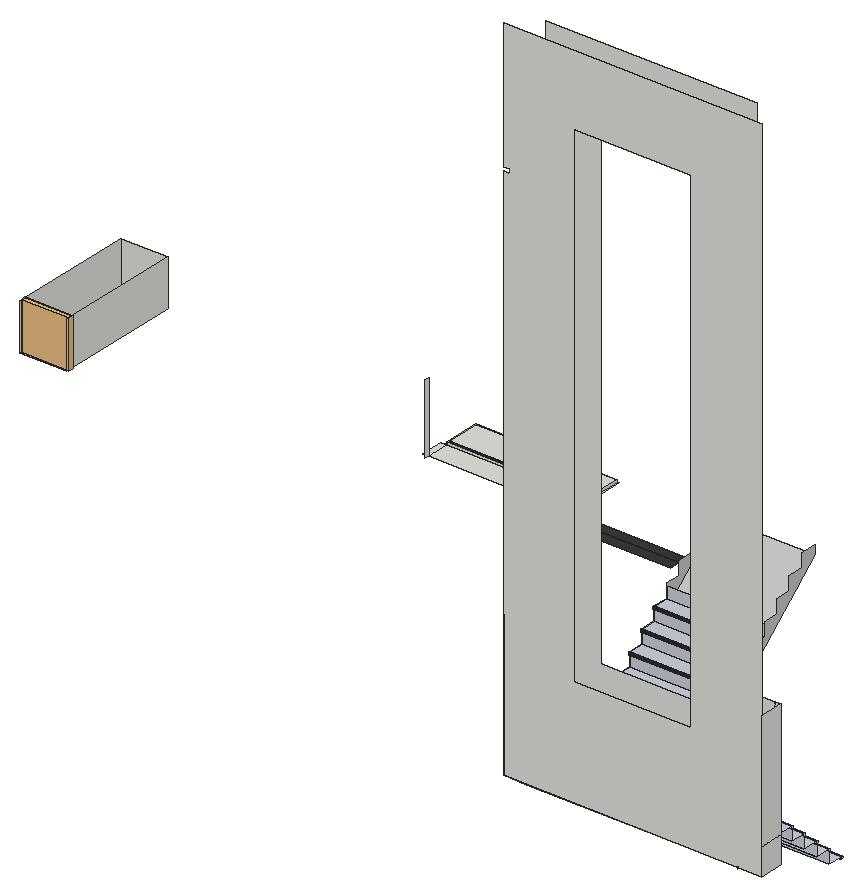
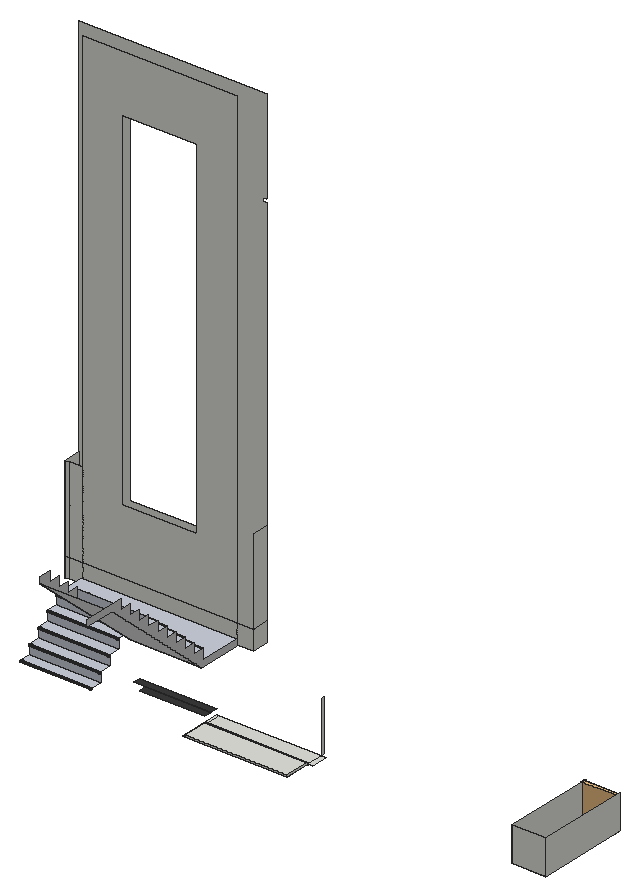
# SketchUp Ruby script. Lengths in inches.
U = 1.inch
M = Sketchup.active_model
def pt(a) = Geom::Point3d.new(a.map { |v| v * U })
def face(e, loops, mat)
  f = e.add_face(loops[0].map { |a| pt(a) })
  loops[1..].each { |l| e.add_face(l.map { |a| pt(a) }).erase! }
  f.material = f.back_material = mat if mat
  f
end
# faces: each face lists its corners as indices into pts; further lists are holes
def faces(e, pts, list, mat = nil) = list.each { |f| face(e, (f[0].is_a?(Array) ? f : [f]).map { |l| l.map { |i| pts[i] } }, mat) }
# xy, xz, yz: faces in a plane at the given z, y or x. An outline is a flat list of corners, or four numbers for a rectangle; further outlines are holes
def ring(l) = l.size == 4 ? [[l[0], l[1]], [l[2], l[1]], [l[2], l[3]], [l[0], l[3]]] : l.each_slice(2).to_a
def flat(e, list, mat, &to3) = list.each { |f| face(e, (f[0].is_a?(Array) ? f : [f]).map { |l| ring(l).map { |u, v| to3.(u, v) } }, mat) }
def xy(e, z, list, mat = nil) = flat(e, list, mat) { |x, y| [x, y, z] }
def xz(e, y, list, mat = nil) = flat(e, list, mat) { |x, z| [x, y, z] }
def yz(e, x, list, mat = nil) = flat(e, list, mat) { |y, z| [x, y, z] }
def lines(e, pts, list) = list.each { |a, b| e.add_line(pt(pts[a]), pt(pts[b])) }
# prism: a flat outline (further loops are holes) pulled along v
def prism(e, loops, v, mat = nil)
  f = face(e, loops, mat); d = Geom::Vector3d.new(v.map { |x| x * U })
  f.pushpull(f.normal.samedirection?(d) ? d.length : -d.length)
end
def box(e, o, s, mat = nil) = prism(e, [[o, [o[0] + s[0], o[1], o[2]], [o[0] + s[0], o[1] + s[1], o[2]], [o[0], o[1] + s[1], o[2]]]], [0, 0, s[2]], mat)
def at(x, y, z, deg = 0) = Geom::Transformation.translation(pt([x, y, z])) * Geom::Transformation.rotation(ORIGIN, Z_AXIS, deg.degrees)
def axes(o, x, y, z) = Geom::Transformation.new([*x, 0, *y, 0, *z, 0, *pt(o).to_a, 1])
def part(name) = M.definitions.add(name)
# library, detail: a bought-in or finely detailed component or shape, given as its bounding box
def library(name, o, s) = part(name).tap { |d| box(d.entities, o, s) }
def detail(e, o, s) = box(e.add_group.entities, o, s)
def put(e, d, t, mat = nil) = e.add_instance(d, t).tap { |i| i.material = mat if mat }
def group(e, t, mat = nil) = e.add_group.tap { |g| g.transformation = t; g.material = mat if mat }.entities
root = M.entities
M.materials.add("[Color M07]").color = [58, 58, 58]
M.materials.add("[Marble Carrara Floor Tile]").color = [204, 208, 219]
M.materials.add("[Polished Concrete New]").color = [200, 200, 203]
c1 = library("Group\#44",[0,0,0],[24.41,3.15,28.35])
xy(root,45.24,[[417.96,89.93,468,90.26]],"[Marble Carrara Floor Tile]")
xy(root,46.4,[[417.96,82.01,468,89.93],[417.96,89.93,468,90.26]],"[Marble Carrara Floor Tile]")
xy(root,52.21,[[417.96,82.01,468,82.34]],"[Marble Carrara Floor Tile]")
xy(root,53.375,[[417.96,74.09,468,82.01],[417.96,82.01,468,82.34]],"[Marble Carrara Floor Tile]")
xy(root,59.18,[[417.96,74.09,468,74.42]],"[Marble Carrara Floor Tile]")
xy(root,60.34,[[417.96,66.17,468,74.09],[417.96,74.09,468,74.42]],"[Marble Carrara Floor Tile]")
xy(root,66.15,[[417.96,66.17,468,66.5]],"[Marble Carrara Floor Tile]")
xy(root,67.32,[[417.96,58.25,468,66.17],[417.96,66.17,468,66.5]],"[Marble Carrara Floor Tile]")
xy(root,69.71,[[359.58,34.49,359.58,66.78,409.62,66.78,409.62,58.25,417.96,58.25,417.96,49.71,468,49.71,468,34.49]],"[Polished Concrete New]")
xy(root,70.4375,[[348,24,360,36],[360,24,468,36],[468,24,477.125,36],[477.125,24,480,36]])
xy(root,73.125,[[417.96,58.25,468,58.58]],"[Marble Carrara Floor Tile]")
xy(root,74.29,[[359.58,34.49,468,34.49,468,58.25,409.62,58.25,409.62,66.17,359.58,66.17],[417.96,58.25,468,58.58]],"[Marble Carrara Floor Tile]")
xy(root,80.1,[[359.58,65.84,409.62,66.17]],"[Marble Carrara Floor Tile]")
xy(root,81.26,[[359.58,65.84,409.62,66.17],[359.58,66.17,409.62,74.09]],"[Marble Carrara Floor Tile]")
xy(root,87.07,[[359.58,73.76,409.62,74.09]],"[Marble Carrara Floor Tile]")
xy(root,88.23,[[359.58,73.76,409.62,74.09],[359.58,74.09,409.62,82.01]],"[Marble Carrara Floor Tile]")
xy(root,94.04,[[359.58,81.68,409.62,82.01]],"[Marble Carrara Floor Tile]")
xy(root,95.2,[[359.58,81.68,409.62,82.01],[359.58,82.01,409.62,89.93]],"[Marble Carrara Floor Tile]")
xy(root,101.01,[[359.58,89.6,409.62,89.93]],"[Marble Carrara Floor Tile]")
xy(root,102.17,[[359.58,89.6,409.62,89.93],[359.58,89.93,409.62,97.85]],"[Marble Carrara Floor Tile]")
xy(root,104,[[286,151,332,156]],"[Color M07]")
xy(root,107.98,[[359.58,97.52,409.62,97.85]],"[Marble Carrara Floor Tile]")
xy(root,108,[[24,120,48,184.5625],[200.9375,156,204,168],[204,156,276,168],[276,156,277.375,168],[203.375,168,204,169.0625],
  [204,168,276,169.0625],[276,168,276.25,169.0625],[203.8125,169.0625,204,186.3125],[204,169.0625,276,186.3125],[276,169.0625,277.1875,186.3125]])
xy(root,108,[[282,151,336,156]],"[Color M07]")
xy(root,109.125,[[204,168,276,169.0625]])
xy(root,109.14,[[359.58,97.52,409.62,97.85],[359.58,97.85,409.62,105.77]],"[Marble Carrara Floor Tile]")
xy(root,109.375,[[204,169.0625,276,186.3125]])
xy(root,114.95,[[359.58,105.4375,409.62,105.77]],"[Marble Carrara Floor Tile]")
xy(root,116.11,[[359.58,105.4375,409.62,105.77],[359.58,105.77,409.62,113.6875]],"[Marble Carrara Floor Tile]")
xz(root,24,[[[348,70.4375,480,70.4375,480,415.2,348,415.2,348,349.2,351,349.2,351,347.2,348,347.2],[384,126,444,379.2]]])
xz(root,34.49,[[359.58,69.71,468,74.29]],"[Polished Concrete New]")
xz(root,36,[[348,70.4375,360,84],[360,70.4375,468,84],[468,70.4375,477.125,84],[477.125,70.4375,480,84],[[360,84,468,415.2],[388,130,440,375.2]],
  [468,84,477.125,144],[477.125,84,480,144]])
xz(root,58.25,[[417.96,67.32,468,73.125],[417.96,73.125,468,74.29]],"[Marble Carrara Floor Tile]")
xz(root,58.25,[[409.62,69.71,417.96,74.29]],"[Polished Concrete New]")
xz(root,66.17,[[417.96,60.34,468,66.15],[417.96,66.15,468,67.32],[359.58,74.29,409.62,80.1],[359.58,80.1,409.62,81.26]],"[Marble Carrara Floor Tile]")
xz(root,74.09,[[417.96,53.375,468,59.18],[417.96,59.18,468,60.34],[359.58,81.26,409.62,87.07],[359.58,87.07,409.62,88.23]],"[Marble Carrara Floor Tile]")
xz(root,82.01,[[417.96,46.4,468,52.21],[417.96,52.21,468,53.375],[359.58,88.23,409.62,94.04],[359.58,94.04,409.62,95.2]],"[Marble Carrara Floor Tile]")
xz(root,89.93,[[417.96,45.24,468,46.4],[359.58,95.2,409.62,101.01],[359.58,101.01,409.62,102.17]],"[Marble Carrara Floor Tile]")
xz(root,97.85,[[359.58,102.17,409.62,107.98],[359.58,107.98,409.62,109.14]],"[Marble Carrara Floor Tile]")
xz(root,105.77,[[359.58,109.14,409.62,114.95],[359.58,114.95,409.62,116.11]],"[Marble Carrara Floor Tile]")
xz(root,113.6875,[[359.58,116.11,409.62,121.92]],"[Marble Carrara Floor Tile]")
xz(root,168,[[204,108,276,109.125]])
xz(root,169.0625,[[204,108,276,109.125],[204,109.125,276,109.375]])
xz(root,184.5625,[[24,108,48,132]])
xz(root,186.3125,[[204,108,276,109.375]])
yz(root,24,[[120,108,184.5625,132]])
yz(root,48,[[120,108,184.5625,132]])
yz(root,204,[[153.875,108,156,144],[168,108,169.0625,109.125],[169.0625,108,186.3125,109.375]])
yz(root,276,[[168,108,169.0625,109.125],[169.0625,108,186.3125,109.375]])
yz(root,348,[[24,70.4375,36,84],[24,84,36,144]])
yz(root,359.58,[[65.84,80.1,65.75,80.12,65.67,80.17,65.6,80.27,65.55,80.39,65.52,80.53,65.51,80.68,65.52,80.83,65.55,80.97,65.6,81.09,65.67,81.18,65.75,81.24,65.84,81.26,66.17,81.26,66.17,80.1],[73.76,87.07,73.67,87.09,73.59,87.15,73.52,87.24,73.47,87.36,73.4375,87.5,73.43,87.65,73.4375,87.8,73.47,87.9375,73.52,88.06,73.59,88.15,73.67,88.21,73.76,88.23,74.09,88.23,74.09,87.07],[81.68,94.04,81.59,94.06,81.51,94.12,81.44,94.21,81.39,94.33,81.36,94.47,81.35,94.62,81.36,94.77,81.39,94.91,81.44,95.03,81.51,95.125,81.59,95.18,81.68,95.2,82.01,95.2,82.01,94.04],[89.6,101.01,89.51,101.03,89.43,101.09,89.36,101.18,89.31,101.3,89.28,101.44,89.27,101.59,89.28,101.74,89.31,101.88,89.36,102,89.43,102.09,89.51,102.15,89.6,102.17,89.93,102.17,89.93,101.01],[97.52,107.98,97.43,108,97.35,108.06,97.28,108.15,97.23,108.27,97.2,108.41,97.1875,108.5625,97.2,108.71,97.23,108.85,97.28,108.97,97.35,109.07,97.43,109.125,97.52,109.14,97.85,109.14,97.85,107.98],
  [105.4375,114.95,105.35,114.97,105.27,115.03,105.2,115.125,105.15,115.24,105.12,115.38,105.11,115.53,105.12,115.68,105.15,115.82,105.2,115.94,105.27,116.04,105.35,116.1,105.4375,116.11,105.77,116.11,105.77,114.95]],"[Marble Carrara Floor Tile]")
yz(root,359.58,[[34.49,69.71,34.49,74.29,66.17,74.29,66.17,81.26,74.09,81.26,74.09,88.23,82.01,88.23,82.01,95.2,89.93,95.2,89.93,102.17,97.85,102.17,97.85,109.14,105.77,109.14,105.77,116.11,113.6875,116.11,113.6875,123.09,121.61,123.09,121.61,130.06,129.53,130.06,129.53,137.03,137.45,137.03,137.45,144,168,144,168,139.43,145.98,139.43,66.78,69.71]],"[Polished Concrete New]")
yz(root,409.62,[[65.84,80.1,66.17,80.1,66.17,81.26,65.84,81.26,65.75,81.24,65.67,81.18,65.6,81.09,65.55,80.97,65.52,80.83,65.51,80.68,65.52,80.53,65.55,80.39,65.6,80.27,65.67,80.17,65.75,80.12],[73.76,87.07,74.09,87.07,74.09,88.23,73.76,88.23,73.67,88.21,73.59,88.15,73.52,88.06,73.47,87.9375,73.4375,87.8,73.43,87.65,73.4375,87.5,73.47,87.36,73.52,87.24,73.59,87.15,73.67,87.09],[81.68,94.04,82.01,94.04,82.01,95.2,81.68,95.2,81.59,95.18,81.51,95.125,81.44,95.03,81.39,94.91,81.36,94.77,81.35,94.62,81.36,94.47,81.39,94.33,81.44,94.21,81.51,94.12,81.59,94.06],[89.6,101.01,89.93,101.01,89.93,102.17,89.6,102.17,89.51,102.15,89.43,102.09,89.36,102,89.31,101.88,89.28,101.74,89.27,101.59,89.28,101.44,89.31,101.3,89.36,101.18,89.43,101.09,89.51,101.03],[97.52,107.98,97.85,107.98,97.85,109.14,97.52,109.14,97.43,109.125,97.35,109.07,97.28,108.97,97.23,108.85,97.2,108.71,97.1875,108.5625,97.2,108.41,97.23,108.27,97.28,108.15,97.35,108.06,97.43,108],
  [105.4375,114.95,105.77,114.95,105.77,116.11,105.4375,116.11,105.35,116.1,105.27,116.04,105.2,115.94,105.15,115.82,105.12,115.68,105.11,115.53,105.12,115.38,105.15,115.24,105.2,115.125,105.27,115.03,105.35,114.97]],"[Marble Carrara Floor Tile]")
yz(root,409.62,[[58.25,69.71,66.78,69.71,145.98,139.43,145.98,144,137.45,144,137.45,137.03,129.53,137.03,129.53,130.06,121.61,130.06,121.61,123.09,113.6875,123.09,113.6875,116.11,105.77,116.11,105.77,109.14,97.85,109.14,97.85,102.17,89.93,102.17,89.93,95.2,82.01,95.2,82.01,88.23,74.09,88.23,74.09,81.26,66.17,81.26,66.17,74.29,58.25,74.29]],"[Polished Concrete New]")
yz(root,417.96,[[89.93,45.24,89.93,46.4,90.26,46.4,90.34,46.38,90.42,46.32,90.49,46.23,90.54,46.11,90.57,45.97,90.59,45.82,90.57,45.67,90.54,45.53,90.49,45.41,90.42,45.32,90.34,45.26,90.26,45.24],[82.01,52.21,82.01,53.375,82.34,53.375,82.42,53.35,82.5,53.3,82.57,53.2,82.62,53.08,82.65,52.94,82.67,52.79,82.65,52.64,82.62,52.5,82.57,52.38,82.5,52.29,82.42,52.23,82.34,52.21],[74.09,59.18,74.09,60.34,74.42,60.34,74.5,60.32,74.58,60.27,74.65,60.17,74.7,60.05,74.73,59.91,74.75,59.76,74.73,59.61,74.7,59.47,74.65,59.35,74.58,59.26,74.5,59.2,74.42,59.18],[66.17,66.15,66.17,67.32,66.5,67.32,66.58,67.3,66.66,67.24,66.73,67.15,66.78,67.03,66.8125,66.89,66.83,66.73,66.8125,66.58,66.78,66.44,66.73,66.32,66.66,66.23,66.58,66.17,66.5,66.15],[58.25,73.125,58.25,74.29,58.58,74.29,58.66,74.27,58.74,74.21,58.81,74.12,58.86,74,58.89,73.86,58.91,73.71,58.89,73.56,58.86,73.42,58.81,73.3,58.74,73.2,58.66,73.15,58.58,73.125]],"[Marble Carrara Floor Tile]")
yz(root,468,[[24,69.71,34.49,70.4375],[34.49,70.4375,36,74.29]])
yz(root,468,[[89.93,45.24,89.93,46.4,90.26,46.4,90.34,46.38,90.42,46.32,90.49,46.23,90.54,46.11,90.57,45.97,90.59,45.82,90.57,45.67,90.54,45.53,90.49,45.41,90.42,45.32,90.34,45.26,90.26,45.24],[82.01,52.21,82.01,53.375,82.34,53.375,82.42,53.35,82.5,53.3,82.57,53.2,82.62,53.08,82.65,52.94,82.67,52.79,82.65,52.64,82.62,52.5,82.57,52.38,82.5,52.29,82.42,52.23,82.34,52.21],[74.09,59.18,74.09,60.34,74.42,60.34,74.5,60.32,74.58,60.27,74.65,60.17,74.7,60.05,74.73,59.91,74.75,59.76,74.73,59.61,74.7,59.47,74.65,59.35,74.58,59.26,74.5,59.2,74.42,59.18],[66.17,66.15,66.17,67.32,66.5,67.32,66.58,67.3,66.66,67.24,66.73,67.15,66.78,67.03,66.8125,66.89,66.83,66.73,66.8125,66.58,66.78,66.44,66.73,66.32,66.66,66.23,66.58,66.17,66.5,66.15],[58.25,73.125,58.25,74.29,58.58,74.29,58.66,74.27,58.74,74.21,58.81,74.12,58.86,74,58.89,73.86,58.91,73.71,58.89,73.56,58.86,73.42,58.81,73.3,58.74,73.2,58.66,73.15,58.58,73.125]],"[Marble Carrara Floor Tile]")
yz(root,480,[[24,70.4375,36,84],[24,84,36,144]])
p = [[468,90.34,45.26],[468,90.26,45.24],[417.96,90.26,45.24],[417.96,90.34,45.26],[468,90.42,45.32],[417.96,90.42,45.32],
  [468,90.49,45.41],[417.96,90.49,45.41],[468,90.54,45.53],[417.96,90.54,45.53],[468,90.57,45.67],[417.96,90.57,45.67],
  [468,90.59,45.82],[417.96,90.59,45.82],[468,90.57,45.97],[417.96,90.57,45.97],[468,90.54,46.11],[417.96,90.54,46.11],
  [468,90.49,46.23],[417.96,90.49,46.23],[468,90.42,46.32],[417.96,90.42,46.32],[468,90.34,46.38],[417.96,90.34,46.38],
  [468,90.26,46.4],[417.96,90.26,46.4],[468,82.42,52.23],[468,82.34,52.21],[417.96,82.34,52.21],[417.96,82.42,52.23],
  [468,82.5,52.29],[417.96,82.5,52.29],[468,82.57,52.38],[417.96,82.57,52.38],[468,82.62,52.5],[417.96,82.62,52.5],
  [468,82.65,52.64],[417.96,82.65,52.64],[468,82.67,52.79],[417.96,82.67,52.79],[468,82.65,52.94],[417.96,82.65,52.94],
  [468,82.62,53.08],[417.96,82.62,53.08],[468,82.57,53.2],[417.96,82.57,53.2],[468,82.5,53.3],[417.96,82.5,53.3],
  [468,82.42,53.35],[417.96,82.42,53.35],[468,82.34,53.375],[417.96,82.34,53.375],[468,74.5,59.2],[468,74.42,59.18],
  [417.96,74.42,59.18],[417.96,74.5,59.2],[468,74.58,59.26],[417.96,74.58,59.26],[468,74.65,59.35],[417.96,74.65,59.35],
  [468,74.7,59.47],[417.96,74.7,59.47],[468,74.73,59.61],[417.96,74.73,59.61],[468,74.75,59.76],[417.96,74.75,59.76],
  [468,74.73,59.91],[417.96,74.73,59.91],[468,74.7,60.05],[417.96,74.7,60.05],[468,74.65,60.17],[417.96,74.65,60.17],
  [468,74.58,60.27],[417.96,74.58,60.27],[468,74.42,60.34],[468,74.5,60.32],[417.96,74.5,60.32],[417.96,74.42,60.34],
  [468,66.58,66.17],[468,66.5,66.15],[417.96,66.5,66.15],[417.96,66.58,66.17],[468,66.66,66.23],[417.96,66.66,66.23],
  [468,66.73,66.32],[417.96,66.73,66.32],[468,66.78,66.44],[417.96,66.78,66.44],[468,66.8125,66.58],[417.96,66.8125,66.58],
  [468,66.83,66.73],[417.96,66.83,66.73],[468,66.8125,66.89],[417.96,66.8125,66.89],[468,66.78,67.03],[417.96,66.78,67.03],
  [468,66.73,67.15],[417.96,66.73,67.15],[468,66.66,67.24],[417.96,66.66,67.24],[468,66.58,67.3],[417.96,66.58,67.3],
  [468,66.5,67.32],[417.96,66.5,67.32],[359.58,66.78,69.71],[359.58,145.98,139.43],[409.62,145.98,139.43],[409.62,66.78,69.71],
  [468,58.66,73.15],[468,58.58,73.125],[417.96,58.58,73.125],[417.96,58.66,73.15],[468,58.74,73.2],[417.96,58.74,73.2],
  [468,58.81,73.3],[417.96,58.81,73.3],[468,58.86,73.42],[417.96,58.86,73.42],[468,58.89,73.56],[417.96,58.89,73.56],
  [468,58.91,73.71],[417.96,58.91,73.71],[468,58.89,73.86],[417.96,58.89,73.86],[468,58.86,74],[417.96,58.86,74],
  [468,58.81,74.12],[417.96,58.81,74.12],[468,58.74,74.21],[417.96,58.74,74.21],[468,58.66,74.27],[417.96,58.66,74.27],
  [468,58.58,74.29],[417.96,58.58,74.29],[359.58,65.67,80.17],[359.58,65.75,80.12],[409.62,65.75,80.12],[409.62,65.67,80.17],
  [359.58,65.84,80.1],[409.62,65.84,80.1],[359.58,65.6,80.27],[409.62,65.6,80.27],[359.58,65.55,80.39],[409.62,65.55,80.39],
  [359.58,65.52,80.53],[409.62,65.52,80.53],[359.58,65.51,80.68],[409.62,65.51,80.68],[359.58,65.52,80.83],[409.62,65.52,80.83],
  [359.58,65.55,80.97],[409.62,65.55,80.97],[359.58,65.6,81.09],[409.62,65.6,81.09],[359.58,65.67,81.18],[409.62,65.67,81.18],
  [359.58,65.75,81.24],[409.62,65.75,81.24],[359.58,65.84,81.26],[409.62,65.84,81.26],[359.58,73.52,87.24],[359.58,73.59,87.15],
  [409.62,73.59,87.15],[409.62,73.52,87.24],[359.58,73.67,87.09],[409.62,73.67,87.09],[359.58,73.76,87.07],[409.62,73.76,87.07],
  [359.58,73.47,87.36],[409.62,73.47,87.36],[359.58,73.4375,87.5],[409.62,73.4375,87.5],[359.58,73.43,87.65],[409.62,73.43,87.65],
  [359.58,73.4375,87.8],[409.62,73.4375,87.8],[359.58,73.47,87.9375],[409.62,73.47,87.9375],[359.58,73.52,88.06],[409.62,73.52,88.06],
  [359.58,73.59,88.15],[409.62,73.59,88.15],[359.58,73.67,88.21],[409.62,73.67,88.21],[359.58,73.76,88.23],[409.62,73.76,88.23],
  [359.58,81.59,94.06],[359.58,81.68,94.04],[409.62,81.68,94.04],[409.62,81.59,94.06],[359.58,81.44,94.21],[359.58,81.51,94.12],
  [409.62,81.51,94.12],[409.62,81.44,94.21],[359.58,81.39,94.33],[409.62,81.39,94.33],[359.58,81.36,94.47],[409.62,81.36,94.47],
  [359.58,81.35,94.62],[409.62,81.35,94.62],[359.58,81.36,94.77],[409.62,81.36,94.77],[359.58,81.39,94.91],[409.62,81.39,94.91],
  [359.58,81.44,95.03],[409.62,81.44,95.03],[359.58,81.51,95.125],[409.62,81.51,95.125],[359.58,81.59,95.18],[409.62,81.59,95.18],
  [359.58,81.68,95.2],[409.62,81.68,95.2],[359.58,89.43,101.09],[359.58,89.51,101.03],[409.62,89.51,101.03],[409.62,89.43,101.09],
  [359.58,89.6,101.01],[409.62,89.6,101.01],[359.58,89.36,101.18],[409.62,89.36,101.18],[359.58,89.31,101.3],[409.62,89.31,101.3],
  [359.58,89.28,101.44],[409.62,89.28,101.44],[359.58,89.27,101.59],[409.62,89.27,101.59],[359.58,89.28,101.74],[409.62,89.28,101.74],
  [359.58,89.31,101.88],[409.62,89.31,101.88],[359.58,89.36,102],[409.62,89.36,102],[359.58,89.43,102.09],[409.62,89.43,102.09],
  [359.58,89.51,102.15],[409.62,89.51,102.15],[359.58,89.6,102.17],[409.62,89.6,102.17],[359.58,97.43,108],[359.58,97.52,107.98],
  [409.62,97.52,107.98],[409.62,97.43,108],[359.58,97.35,108.06],[409.62,97.35,108.06],[359.58,97.28,108.15],[409.62,97.28,108.15],
  [359.58,97.23,108.27],[409.62,97.23,108.27],[359.58,97.2,108.41],[409.62,97.2,108.41],[359.58,97.1875,108.5625],[409.62,97.1875,108.5625],
  [359.58,97.2,108.71],[409.62,97.2,108.71],[359.58,97.23,108.85],[409.62,97.23,108.85],[359.58,97.28,108.97],[409.62,97.28,108.97],
  [359.58,97.35,109.07],[409.62,97.35,109.07],[359.58,97.43,109.125],[409.62,97.43,109.125],[359.58,97.52,109.14],[409.62,97.52,109.14],
  [359.58,105.2,115.125],[359.58,105.27,115.03],[409.62,105.27,115.03],[409.62,105.2,115.125],[359.58,105.35,114.97],[409.62,105.35,114.97],
  [359.58,105.4375,114.95],[409.62,105.4375,114.95],[359.58,105.15,115.24],[409.62,105.15,115.24],[359.58,105.12,115.38],[409.62,105.12,115.38],
  [359.58,105.11,115.53],[409.62,105.11,115.53],[359.58,105.12,115.68],[409.62,105.12,115.68],[359.58,105.15,115.82],[409.62,105.15,115.82],
  [359.58,105.2,115.94],[409.62,105.2,115.94],[359.58,105.27,116.04],[409.62,105.27,116.04],[359.58,105.35,116.1],[409.62,105.35,116.1],
  [359.58,105.4375,116.11],[409.62,105.4375,116.11]]
faces(root,p,[[0,1,2,3],[4,0,3,5],[6,4,5,7],[8,6,7,9],[10,8,9,11],[12,10,11,13],[14,12,13,15],[16,14,15,17],
  [18,16,17,19],[20,18,19,21],[22,20,21,23],[24,22,23,25],[26,27,28,29],[30,26,29,31],[32,30,31,33],[34,32,33,35],
  [36,34,35,37],[38,36,37,39],[40,38,39,41],[42,40,41,43],[44,42,43,45],[46,44,45,47],[48,46,47,49],[50,48,49,51],
  [52,53,54,55],[56,52,55,57],[58,56,57,59],[60,58,59,61],[62,60,61,63],[64,62,63,65],[66,64,65,67],[68,66,67,69],
  [70,68,69,71],[72,70,71,73],[74,75,76,77],[75,72,73,76],[78,79,80,81],[82,78,81,83],[84,82,83,85],[86,84,85,87],
  [88,86,87,89],[90,88,89,91],[92,90,91,93],[94,92,93,95],[96,94,95,97],[98,96,97,99],[100,98,99,101],[102,100,101,103],
  [108,109,110,111],[112,108,111,113],[114,112,113,115],[116,114,115,117],[118,116,117,119],[120,118,119,121],[122,120,121,123],[124,122,123,125],
  [126,124,125,127],[128,126,127,129],[130,128,129,131],[132,130,131,133],[134,135,136,137],[135,138,139,136],[140,134,137,141],[142,140,141,143],
  [144,142,143,145],[146,144,145,147],[148,146,147,149],[150,148,149,151],[152,150,151,153],[154,152,153,155],[156,154,155,157],[158,156,157,159],
  [160,161,162,163],[161,164,165,162],[164,166,167,165],[168,160,163,169],[170,168,169,171],[172,170,171,173],[174,172,173,175],[176,174,175,177],
  [178,176,177,179],[180,178,179,181],[182,180,181,183],[184,182,183,185],[186,187,188,189],[190,191,192,193],[191,186,189,192],[194,190,193,195],
  [196,194,195,197],[198,196,197,199],[200,198,199,201],[202,200,201,203],[204,202,203,205],[206,204,205,207],[208,206,207,209],[210,208,209,211],
  [212,213,214,215],[213,216,217,214],[218,212,215,219],[220,218,219,221],[222,220,221,223],[224,222,223,225],[226,224,225,227],[228,226,227,229],
  [230,228,229,231],[232,230,231,233],[234,232,233,235],[236,234,235,237],[238,239,240,241],[242,238,241,243],[244,242,243,245],[246,244,245,247],
  [248,246,247,249],[250,248,249,251],[252,250,251,253],[254,252,253,255],[256,254,255,257],[258,256,257,259],[260,258,259,261],[262,260,261,263],
  [264,265,266,267],[265,268,269,266],[268,270,271,269],[272,264,267,273],[274,272,273,275],[276,274,275,277],[278,276,277,279],[280,278,279,281],
  [282,280,281,283],[284,282,283,285],[286,284,285,287],[288,286,287,289]],"[Marble Carrara Floor Tile]")
faces(root,p,[[104,105,106,107]],"[Polished Concrete New]")
put(root,c1,axes([24,120.78,108],[0.9975,0,0],[0,0.75,0],[0,0,0.8484]))
